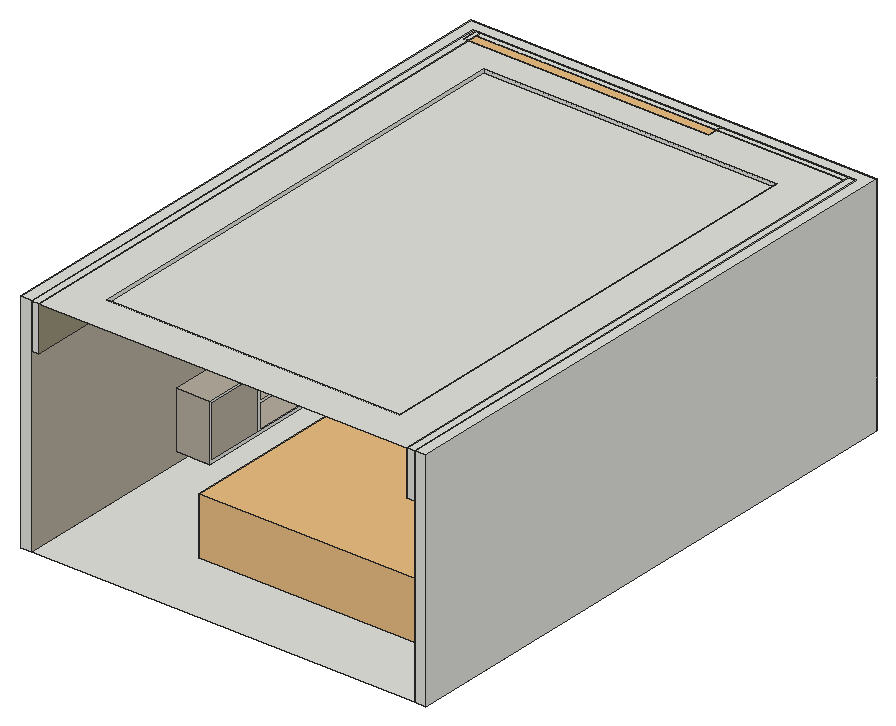
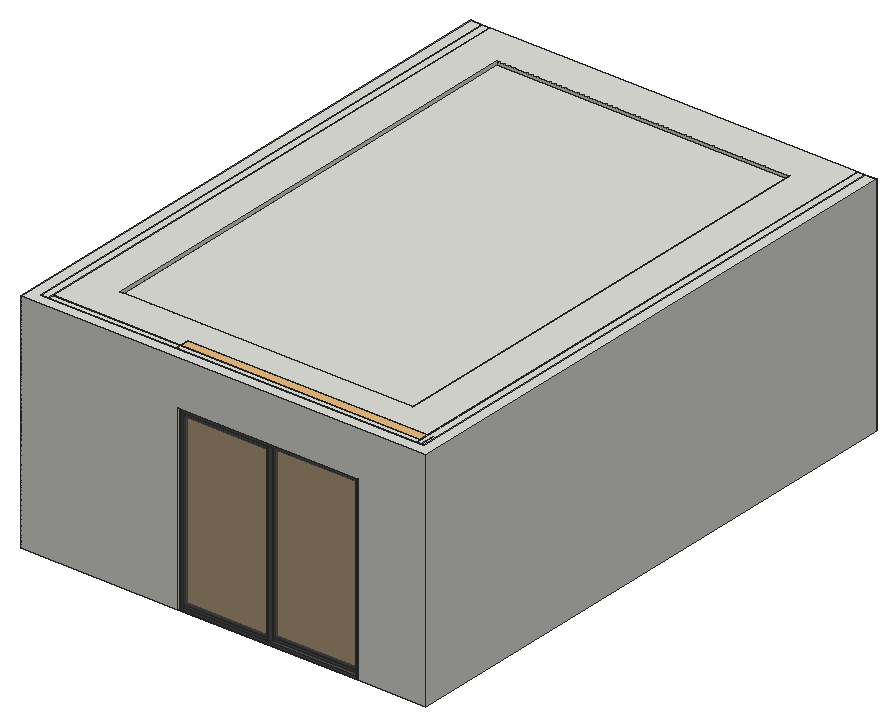
# SketchUp Ruby script. Lengths in inches.
U = 1.inch
M = Sketchup.active_model
def pt(a) = Geom::Point3d.new(a.map { |v| v * U })
def face(e, loops, mat)
  f = e.add_face(loops[0].map { |a| pt(a) })
  loops[1..].each { |l| e.add_face(l.map { |a| pt(a) }).erase! }
  f.material = f.back_material = mat if mat
  f
end
# faces: each face lists its corners as indices into pts; further lists are holes
def faces(e, pts, list, mat = nil) = list.each { |f| face(e, (f[0].is_a?(Array) ? f : [f]).map { |l| l.map { |i| pts[i] } }, mat) }
# xy, xz, yz: faces in a plane at the given z, y or x. An outline is a flat list of corners, or four numbers for a rectangle; further outlines are holes
def ring(l) = l.size == 4 ? [[l[0], l[1]], [l[2], l[1]], [l[2], l[3]], [l[0], l[3]]] : l.each_slice(2).to_a
def flat(e, list, mat, &to3) = list.each { |f| face(e, (f[0].is_a?(Array) ? f : [f]).map { |l| ring(l).map { |u, v| to3.(u, v) } }, mat) }
def xy(e, z, list, mat = nil) = flat(e, list, mat) { |x, y| [x, y, z] }
def xz(e, y, list, mat = nil) = flat(e, list, mat) { |x, z| [x, y, z] }
def yz(e, x, list, mat = nil) = flat(e, list, mat) { |y, z| [x, y, z] }
def lines(e, pts, list) = list.each { |a, b| e.add_line(pt(pts[a]), pt(pts[b])) }
# prism: a flat outline (further loops are holes) pulled along v
def prism(e, loops, v, mat = nil)
  f = face(e, loops, mat); d = Geom::Vector3d.new(v.map { |x| x * U })
  f.pushpull(f.normal.samedirection?(d) ? d.length : -d.length)
end
def box(e, o, s, mat = nil) = prism(e, [[o, [o[0] + s[0], o[1], o[2]], [o[0] + s[0], o[1] + s[1], o[2]], [o[0], o[1] + s[1], o[2]]]], [0, 0, s[2]], mat)
def at(x, y, z, deg = 0) = Geom::Transformation.translation(pt([x, y, z])) * Geom::Transformation.rotation(ORIGIN, Z_AXIS, deg.degrees)
def axes(o, x, y, z) = Geom::Transformation.new([*x, 0, *y, 0, *z, 0, *pt(o).to_a, 1])
def part(name) = M.definitions.add(name)
# library, detail: a bought-in or finely detailed component or shape, given as its bounding box
def library(name, o, s) = part(name).tap { |d| box(d.entities, o, s) }
def detail(e, o, s) = box(e.add_group.entities, o, s)
def put(e, d, t, mat = nil) = e.add_instance(d, t).tap { |i| i.material = mat if mat }
def group(e, t, mat = nil) = e.add_group.tap { |g| g.transformation = t; g.material = mat if mat }.entities
root = M.entities
M.materials.add("[0135_DarkGray]").color = [81, 81, 81]
M.materials.add("[Color_008]").color = [30, 30, 30]
M.materials.add("[Color_B19]").color = [180, 172, 158]
M.materials.add("[Color_D15]").color = [153, 145, 122]
M.materials.add("[Translucent Glass Gray]").color = [128, 128, 128]
M.materials["[Translucent Glass Gray]"].alpha = 0.15
c1 = part("PENTEK_RP Fineline 50S_Sliding_DoorCase_E1")
box(c1.entities,[0,0,0],[1.51,3.66,99.27],"[0135_DarkGray]")
c2 = part("PENTEK_RP Fineline 50S_SlidingDooe_Case_E2")
box(c2.entities,[0,0,0],[96.25,3.66,1.51],"[0135_DarkGray]")
c3 = part("pentek_RP Fineline 50S_SlidingDoor_Case")
put(c3.entities,c1,at(97.76,0,0))
put(c3.entities,c2,at(1.51,0,0))
put(c3.entities,c1,at(0,0,0))
put(c3.entities,c2,at(1.51,0,97.76))
c4 = part("PENTEK_RP Fineline 50S_SlidingDoor_GlazingBead_2")
box(c4.entities,[0,0,0],[0.56,0.59,94.39],"[0135_DarkGray]")
c5 = part("PENTEK_RP Fineline 50S_SlidingDoor_Glass")
box(c5.entities,[0,0,0],[46.58,0.16,94.39],"[Translucent Glass Gray]")
c6 = part("PENTEK_RP Fineline 50S_SlidingDoor_GlazingBead")
box(c6.entities,[0,0,0],[45.47,0.59,0.56],"[0135_DarkGray]")
c7 = part("PENTEK_RP Fineline 50S_SlidingDoor_Leaf_E1")
xy(c7.entities,0,[[0,0,0.93,1.97],[0.93,1.57,1.49,1.97]],"[0135_DarkGray]")
xy(c7.entities,96.25,[[0,0,0.93,0,0.93,1.57,1.49,1.57,1.49,1.97,0,1.97]],"[0135_DarkGray]")
xz(c7.entities,0,[[0,0,0.93,96.25]],"[0135_DarkGray]")
xz(c7.entities,1.57,[[0.93,0,1.49,95.32],[0.93,95.32,1.49,96.25]],"[0135_DarkGray]")
xz(c7.entities,1.97,[[0,0,1.49,96.25]],"[0135_DarkGray]")
yz(c7.entities,0,[[0,0,1.97,96.25]],"[0135_DarkGray]")
yz(c7.entities,0.93,[[0,0,1.57,0.93],[0,0.93,1.57,95.32],[0,95.32,1.57,96.25]],"[0135_DarkGray]")
yz(c7.entities,1.49,[[1.57,0,1.97,95.32],[1.57,95.32,1.97,96.25]],"[0135_DarkGray]")
c8 = part("PENTEK_RP Fineline 50S_SlidingDoor_Leaf_E2")
xy(c8.entities,0,[[0,0,0,1.57,0.56,1.57,0.56,1.97,46.02,1.97,46.02,1.57,46.58,1.57,46.58,0]],"[0135_DarkGray]")
xy(c8.entities,0.93,[[0,0,46.58,1.57]],"[0135_DarkGray]")
xy(c8.entities,1.49,[[0.56,1.57,46.02,1.97]],"[0135_DarkGray]")
xz(c8.entities,0,[[0,0,46.58,0.93]],"[0135_DarkGray]")
xz(c8.entities,1.57,[[0,0,0.56,0.93],[46.02,0,46.58,0.93],[0.56,0.93,46.02,1.49]],"[0135_DarkGray]")
xz(c8.entities,1.97,[[0.56,0,46.02,1.49]],"[0135_DarkGray]")
yz(c8.entities,0,[[0,0,1.57,0.93]],"[0135_DarkGray]")
yz(c8.entities,0.56,[[1.57,0,1.97,0.93],[1.57,0.93,1.97,1.49]],"[0135_DarkGray]")
yz(c8.entities,46.02,[[1.57,0,1.97,0.93],[1.57,0.93,1.97,1.49]],"[0135_DarkGray]")
yz(c8.entities,46.58,[[0,0,1.57,0.93]],"[0135_DarkGray]")
c9 = part("PENTEK_RP Fineline S_SlidingDoor_Leaf1")
put(c9.entities,c4,at(0.93,0,0.93))
put(c9.entities,c4,at(46.96,0,0.93))
put(c9.entities,c5,at(1.49,1.42,0.93))
put(c9.entities,c6,at(1.49,0,0.93))
put(c9.entities,c5,at(1.49,0.59,0.93))
put(c9.entities,c7,at(0,0,0))
put(c9.entities,c7,axes([48.44,0,0],[-1,0,0],[0,1,0],[0,0,1]))
put(c9.entities,c8,axes([0.93,0,96.25],[1,0,0],[0,1,0],[0,0,-1]))
put(c9.entities,c8,at(0.93,0,0))
put(c9.entities,c6,at(1.49,0,94.77))
c10 = part("PENTEK_RP Fineline 50S_SlidingDoor_Leaf2")
put(c10.entities,c5,at(1.49,1.42,0.93))
put(c10.entities,c6,at(1.49,0,94.77))
put(c10.entities,c4,at(46.96,0,0.93))
put(c10.entities,c5,at(1.49,0.59,0.93))
put(c10.entities,c4,at(0.93,0,0.93))
put(c10.entities,c7,at(0,0,0))
put(c10.entities,c7,axes([48.44,0,0],[-1,0,0],[0,1,0],[0,0,1]))
put(c10.entities,c6,at(1.49,0,0.93))
put(c10.entities,c8,axes([0.93,0,96.25],[1,0,0],[0,1,0],[0,0,-1]))
put(c10.entities,c8,at(0.93,0,0))
c11 = library("Sofa+Set+3+(1)\#1",[-143.38,0,-0.17],[143.38,111.7,30.39])
c12 = library("Garniza_zaclona\#2",[1.52,0,0],[127.96,8.15,78.72])
c13 = library("Group\#48",[0,-0.16,0],[10.12,10.28,9.06])
xy(root,142.975,[[1271.106,0,1277.106,60],[1277.106,0,1481.106,0,1481.106,276,1409.106,276,1409.106,294,1403.106,294,1403.106,300,1307.106,300,1307.106,294,1277.106,294],[1481.106,0,1487.106,60]])
xy(root,148.975,[[1277.106,96,1295.106,192]])
xy(root,149.975,[[1294.926,97,1295.106,128.333],[1294.926,159.667,1295.106,191]])
xy(root,150.175,[[1294.926,97.2,1295.106,128.133],[1294.926,159.867,1295.106,190.8]])
xy(root,150.975,[[1277.106,129.333,1295.106,158.667]],"[Color_B19]")
xy(root,163.475,[[1277.106,129.333,1295.106,158.667]],"[Color_B19]")
xy(root,164.475,[[1277.106,129.333,1295.106,158.667]],"[Color_B19]")
xy(root,176.975,[[1277.106,129.333,1295.106,158.667]],"[Color_B19]")
xy(root,177.775,[[1294.926,97.2,1295.106,128.133],[1294.926,159.867,1295.106,190.8]])
xy(root,177.975,[[1294.926,97,1295.106,128.333],[1294.926,159.667,1295.106,191]])
xy(root,178.975,[[1277.106,96,1295.106,192]],"[Color_B19]")
xy(root,179.975,[[1410.106,276,1456.106,294],[1457.106,276,1480.106,294]])
xy(root,198.475,[[1457.106,276,1480.106,294]])
xy(root,199.475,[[1457.106,276,1480.106,294]])
xy(root,218.475,[[1457.106,276,1480.106,294]])
xy(root,219.475,[[1457.106,276,1480.106,294]])
xy(root,237.975,[[1410.106,276,1456.106,294],[1457.106,276,1480.106,294]])
xy(root,238.975,[[1277.106,0,1281.106,294],[1477.106,0,1481.106,276],[1409.106,276,1477.106,291],[1477.106,276,1481.106,294],[1281.106,291,1307.106,294],
  [1307.106,291,1403.106,294],[1403.106,291,1409.106,294],[1409.106,291,1477.106,294],[1307.106,294,1403.106,300]])
xy(root,262.975,[[1271.106,0,1277.106,0,1277.106,294,1481.106,294,1481.106,0,1487.106,0,1487.106,300,1271.106,300],[1277.106,0,1281.106,294],[1477.106,0,1481.106,294],[1281.106,291,1477.106,294]])
xz(root,0,[[1271.106,142.975,1277.106,262.975],[1481.106,142.975,1487.106,262.975],[1277.106,238.975,1281.106,262.975],[1477.106,238.975,1481.106,262.975]])
xz(root,96,[[1277.106,148.975,1295.106,178.975]],"[Color_B19]")
xz(root,97,[[1294.926,149.975,1295.106,177.975]])
xz(root,97.2,[[1294.926,150.175,1295.106,177.775]])
xz(root,128.133,[[1294.926,150.175,1295.106,177.775]])
xz(root,128.333,[[1294.926,149.975,1295.106,177.975]])
xz(root,129.333,[[1277.106,150.975,1295.106,162.85],[1277.106,162.85,1295.106,162.975],[1277.106,162.975,1295.106,163.475],[1277.106,164.475,1295.106,164.975],[1277.106,164.975,1295.106,176.975]])
xz(root,158.667,[[1277.106,162.975,1295.106,163.475],[1277.106,164.475,1295.106,164.975]])
xz(root,158.667,[[1277.106,150.975,1295.106,162.975],[1277.106,164.975,1295.106,176.975]],"[Color_B19]")
xz(root,159.667,[[1294.926,149.975,1295.106,177.975]])
xz(root,159.867,[[1294.926,150.175,1295.106,177.775]])
xz(root,190.8,[[1294.926,150.175,1295.106,177.775]])
xz(root,191,[[1294.926,149.975,1295.106,177.975]])
xz(root,192,[[1277.106,148.975,1295.106,178.975]])
xz(root,276,[[[1409.106,142.975,1410.106,142.975,1410.106,178.975,1481.106,178.975,1481.106,238.975,1409.106,238.975],[1410.106,179.975,1456.106,237.975],[1457.106,199.475,1480.106,218.475],[1457.106,179.975,1480.106,198.475],[1457.106,219.475,1480.106,237.975]],[1410.106,142.975,1481.106,178.975]])
xz(root,291,[[1281.106,238.975,1477.106,262.975]],"[Color_D15]")
xz(root,294,[[1277.106,142.975,1307.106,238.975],[1403.106,142.975,1409.106,238.975],[1457.106,179.975,1480.106,198.475],[1457.106,199.475,1480.106,218.475],[1457.106,219.475,1480.106,237.975],
  [1277.106,238.975,1281.106,262.975],[1281.106,238.975,1477.106,262.975],[1477.106,238.975,1481.106,262.975]])
xz(root,294,[[1410.106,179.975,1456.106,237.975]],"[Color_B19]")
xz(root,300,[[1271.106,142.975,1271.106,262.975,1487.106,262.975,1487.106,142.975,1403.106,142.975,1403.106,238.975,1307.106,238.975,1307.106,142.975]])
yz(root,1271.106,[[0,142.975,300,262.975]])
yz(root,1277.106,[[0,238.975,294,262.975]])
yz(root,1277.106,[[[0,142.975,294,238.975],[96,148.975,192,178.975]],[129.333,150.975,158.667,163.475],[129.333,164.475,158.667,176.975]],"[Color_B19]")
yz(root,1281.106,[[291,238.975,294,262.975]])
yz(root,1281.106,[[0,238.975,291,262.975]],"[Color_D15]")
yz(root,1294.926,[[[97,149.975,128.333,177.975],[97.2,150.175,128.133,177.775]],[[159.667,149.975,191,177.975],[159.867,150.175,190.8,177.775]]])
yz(root,1295.106,[[[96,148.975,192,178.975],[97,149.975,191,177.975]],[[128.333,149.975,159.667,177.975],[129.333,150.975,158.667,163.475],[129.333,164.475,158.667,176.975]]])
yz(root,1295.106,[[97.2,150.175,128.133,177.775],[159.867,150.175,190.8,177.775]],"[Color_B19]")
yz(root,1307.106,[[294,142.975,300,238.975]])
yz(root,1403.106,[[294,142.975,300,238.975]])
yz(root,1409.106,[[276,142.975,294,238.975]])
yz(root,1410.106,[[276,179.975,294,237.975]])
yz(root,1456.106,[[276,179.975,294,218.975],[276,218.975,294,237.975]])
yz(root,1457.106,[[276,179.975,294,198.475],[276,199.475,294,218.475],[276,219.475,294,237.975]])
yz(root,1477.106,[[291,238.975,294,262.975]])
yz(root,1477.106,[[0,238.975,291,262.975]],"[Color_B19]")
yz(root,1480.106,[[276,179.975,294,198.475],[276,199.475,294,218.475],[276,219.475,294,237.975]])
yz(root,1481.106,[[0,238.975,294,262.975]])
yz(root,1481.106,[[0,142.975,276,238.975]],"[Color_B19]")
yz(root,1487.106,[[0,142.975,300,262.975]])
p = [[1424.036,-355.269,847.505],[1424.038,-355.27,847.505],[1424.038,-355.27,848.541],[1424.036,-355.269,848.541],[1656.68,-603.859,682.345],[1656.678,-603.859,682.345],
  [1656.678,-603.859,681.309],[1656.68,-603.859,681.309],[1534.924,-292.551,627.597],[1534.922,-292.551,627.597],[1534.922,-292.551,626.561],[1534.924,-292.551,626.561],
  [1937.164,-66.977,642.226],[1937.162,-66.976,642.226],[1937.162,-66.976,641.19],[1937.164,-66.977,641.19]]
lines(root,p,[[0,1],[2,3],[4,5],[6,7],[8,9],[10,11],[12,13],[14,15]])
g1 = group(root,at(1307.11,295.72,142.97))
put(g1,c3,axes([0,0.39,0],[0.96704,0,0],[0,1,0],[0,0,0.96704]))
put(g1,c9,axes([1.46,0,1.46],[0.96704,0,0],[0,1,0],[0,0,0.96704]))
put(g1,c10,axes([47.69,1.97,1.46],[0.96704,0,0],[0,1,0],[0,0,0.96704]))
put(root,c11,axes([1334.36,39.83,143.14],[0,-1.27,0],[1.23,0,0],[0,0,1]))
put(root,c12,axes([1277.11,285.85,142.97],[1.01949,0,0],[0,1,0],[0,0,1.52445]))
g2 = group(root,at(1282.11,176.89,192.25),"[Color_008]")
xy(g2,0,[[-2,-70.79,0,0]])
xy(g2,18.18,[[-5,-43.72,-2,-30.28]])
xy(g2,24.43,[[-5,-43.72,-2,-30.28]])
xy(g2,43.75,[[-2,-70.79,0,0]])
xz(g2,-70.79,[[-2,0,0,43.75]])
xz(g2,-43.72,[[-5,18.18,-2,24.43]])
xz(g2,-30.28,[[-5,18.18,-2,24.43]])
xz(g2,0,[[-2,0,0,43.75]])
yz(g2,-5,[[-43.72,18.18,-30.28,24.43]])
yz(g2,-2,[[[-70.79,0,0,43.75],[-43.72,18.18,-30.28,24.43]]])
yz(g2,0,[[-70.79,0,0,43.75]])
g3 = group(root,at(1281.11,0,262.97))
xy(g3,-2,[[18,18,178,20],[18,20,20,273],[20,20,176,271],[176,20,178,273],[20,271,176,273]])
xy(g3,0,[[[0,0,196,291],[20,20,176,271]]])
xz(g3,18,[[18,-6,178,-2]])
xz(g3,20,[[20,-2,176,0]])
xz(g3,271,[[20,-2,176,0]])
xz(g3,273,[[18,-6,178,-2]])
yz(g3,18,[[18,-6,273,-2]])
yz(g3,20,[[20,-2,271,0]])
yz(g3,176,[[20,-2,271,0]])
yz(g3,178,[[18,-6,273,-2]])
g4 = group(g3,at(18,18,-15.06))
xy(g4,9.06,[[0,0,160,255]])
put(g4,c13,axes([143.47,16.84,9.06],[-1,0,0],[0,1,0],[0,0,-1]))
put(g4,c13,axes([143.47,225.21,9.06],[-1,0,0],[0,1,0],[0,0,-1]))
put(g4,c13,axes([143.47,114.09,9.06],[-1,0,0],[0,1,0],[0,0,-1]))
put(g4,c13,axes([24.22,16.84,9.06],[-1,0,0],[0,1,0],[0,0,-1]))
put(g4,c13,axes([24.22,225.21,9.06],[-1,0,0],[0,1,0],[0,0,-1]))
put(g4,c13,axes([24.22,114.09,9.06],[-1,0,0],[0,1,0],[0,0,-1]))
put(g4,c13,axes([83.16,225.21,9.06],[-1,0,0],[0,1,0],[0,0,-1]))
put(g4,c13,axes([83.16,16.84,9.06],[-1,0,0],[0,1,0],[0,0,-1]))
